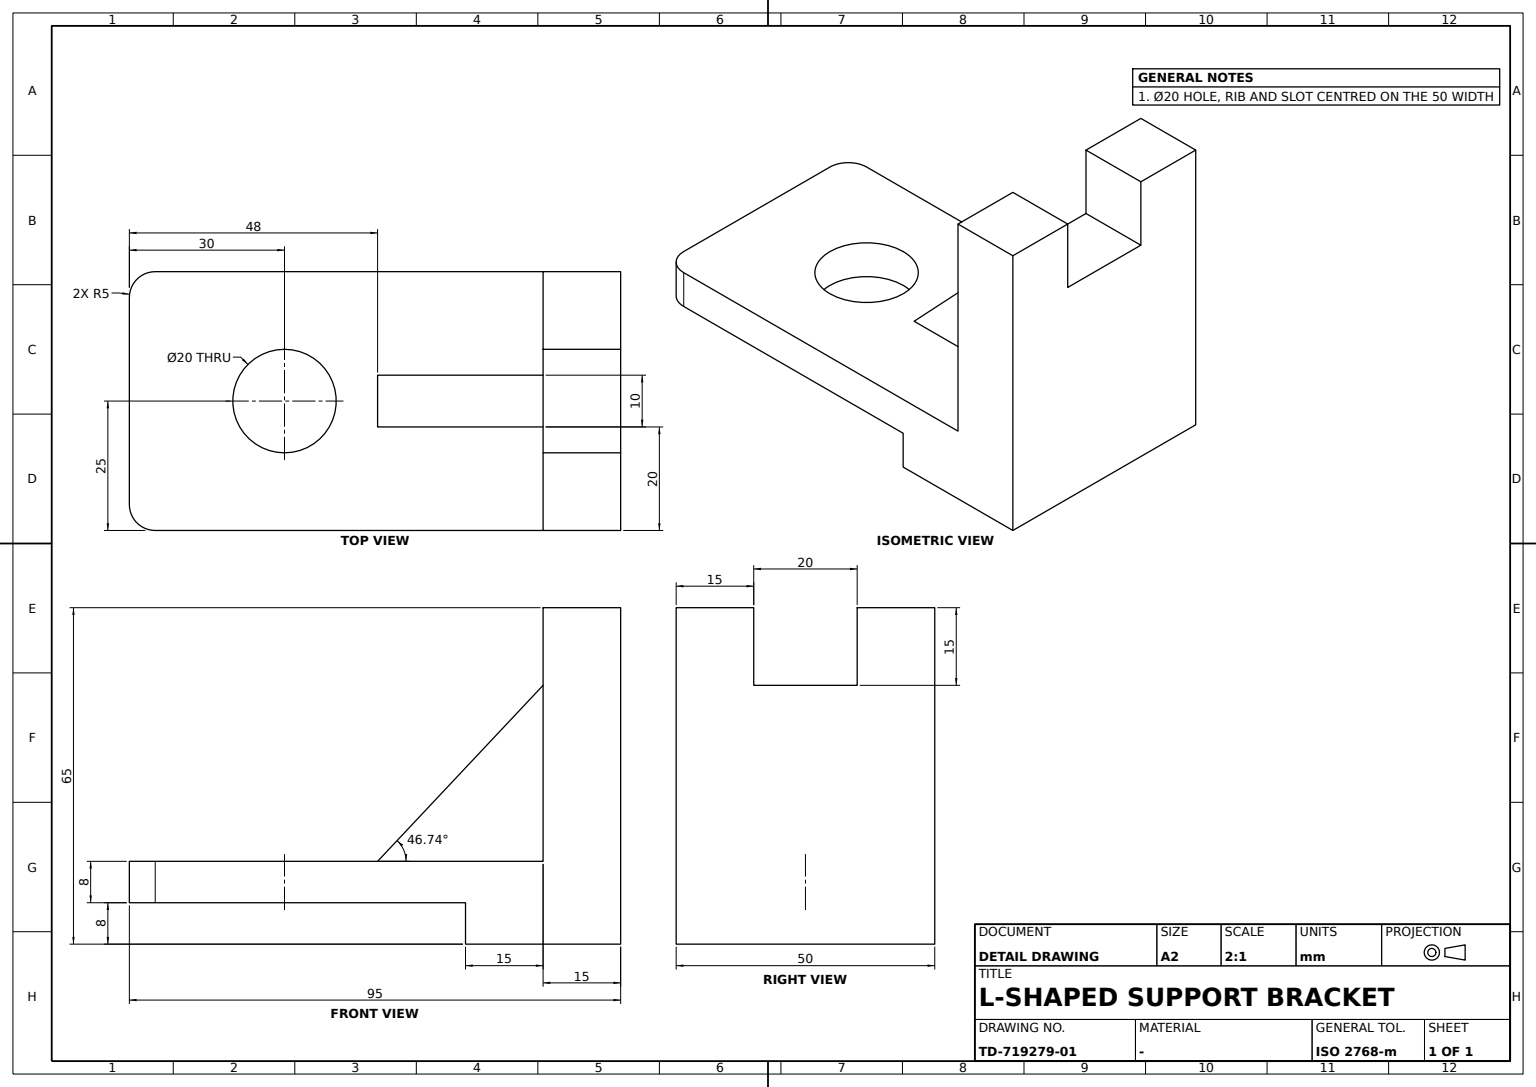
ISO-10303-21;
HEADER;
FILE_DESCRIPTION((''),'2;1');
FILE_NAME('','',(''),(''),'','','');
FILE_SCHEMA(('AUTOMOTIVE_DESIGN'));
ENDSEC;
DATA;
#1=APPLICATION_CONTEXT('');
#2=PRODUCT_CONTEXT('',#1,'mechanical');
#3=PRODUCT('','','',(#2));
#4=PRODUCT_DEFINITION_FORMATION('','',#3);
#5=PRODUCT_DEFINITION_CONTEXT('',#1,'design');
#6=PRODUCT_DEFINITION('','',#4,#5);
#7=PRODUCT_DEFINITION_SHAPE('','',#6);
#8=(LENGTH_UNIT()NAMED_UNIT(*)SI_UNIT(.MILLI.,.METRE.));
#9=(NAMED_UNIT(*)PLANE_ANGLE_UNIT()SI_UNIT($,.RADIAN.));
#10=(NAMED_UNIT(*)SI_UNIT($,.STERADIAN.)SOLID_ANGLE_UNIT());
#11=UNCERTAINTY_MEASURE_WITH_UNIT(LENGTH_MEASURE(0.005),#8,'distance_accuracy_value','');
#12=(GEOMETRIC_REPRESENTATION_CONTEXT(3)GLOBAL_UNCERTAINTY_ASSIGNED_CONTEXT((#11))GLOBAL_UNIT_ASSIGNED_CONTEXT((#8,#9,#10))REPRESENTATION_CONTEXT('',''));
#13=CARTESIAN_POINT('',(-5.,-47.,16.));
#14=VERTEX_POINT('',#13);
#15=CARTESIAN_POINT('',(-5.,-15.,16.));
#16=VERTEX_POINT('',#15);
#17=CARTESIAN_POINT('',(-5.,0.,16.));
#18=DIRECTION('',(0.,1.,0.));
#19=VECTOR('',#18,1000.);
#20=LINE('',#17,#19);
#21=EDGE_CURVE('',#14,#16,#20,.T.);
#22=ORIENTED_EDGE('',*,*,#21,.F.);
#23=CARTESIAN_POINT('',(-5.,-15.,50.));
#24=VERTEX_POINT('',#23);
#25=DIRECTION('',(0.,0.685364699,0.728199993));
#26=VECTOR('',#25,1000.);
#27=LINE('',#13,#26);
#28=EDGE_CURVE('',#14,#24,#27,.T.);
#29=ORIENTED_EDGE('',*,*,#28,.T.);
#30=CARTESIAN_POINT('',(-5.,-15.,0.));
#31=DIRECTION('',(0.,0.,1.));
#32=VECTOR('',#31,1000.);
#33=LINE('',#30,#32);
#34=EDGE_CURVE('',#16,#24,#33,.T.);
#35=ORIENTED_EDGE('',*,*,#34,.F.);
#36=EDGE_LOOP('',(#22,#29,#35));
#37=FACE_BOUND('',#36,.T.);
#38=CARTESIAN_POINT('',(-5.,0.,0.));
#39=DIRECTION('',(-1.,0.,0.));
#40=AXIS2_PLACEMENT_3D('',#38,#39,#31);
#41=PLANE('',#40);
#42=ADVANCED_FACE('',(#37),#41,.T.);
#43=CARTESIAN_POINT('',(20.,-95.,8.));
#44=VERTEX_POINT('',#43);
#45=CARTESIAN_POINT('',(-20.,-95.,8.));
#46=VERTEX_POINT('',#45);
#47=CARTESIAN_POINT('',(25.,-95.,8.));
#48=VECTOR('',#39,1000.);
#49=LINE('',#47,#48);
#50=EDGE_CURVE('',#44,#46,#49,.T.);
#51=ORIENTED_EDGE('',*,*,#50,.F.);
#52=CARTESIAN_POINT('',(20.,-95.,16.));
#53=VERTEX_POINT('',#52);
#54=LINE('',#52,#32);
#55=EDGE_CURVE('',#44,#53,#54,.T.);
#56=ORIENTED_EDGE('',*,*,#55,.T.);
#57=CARTESIAN_POINT('',(-20.,-95.,16.));
#58=VERTEX_POINT('',#57);
#59=CARTESIAN_POINT('',(25.,-95.,16.));
#60=LINE('',#59,#48);
#61=EDGE_CURVE('',#53,#58,#60,.T.);
#62=ORIENTED_EDGE('',*,*,#61,.T.);
#63=DIRECTION('',(0.,0.,-1.));
#64=VECTOR('',#63,1000.);
#65=LINE('',#57,#64);
#66=EDGE_CURVE('',#58,#46,#65,.T.);
#67=ORIENTED_EDGE('',*,*,#66,.T.);
#68=EDGE_LOOP('',(#51,#56,#62,#67));
#69=FACE_BOUND('',#68,.T.);
#70=AXIS2_PLACEMENT_3D('',#59,#18,#31);
#71=PLANE('',#70);
#72=ADVANCED_FACE('',(#69),#71,.F.);
#73=CARTESIAN_POINT('',(-25.,0.,65.));
#74=VERTEX_POINT('',#73);
#75=CARTESIAN_POINT('',(-25.,-15.,65.));
#76=VERTEX_POINT('',#75);
#77=DIRECTION('',(0.,-1.,0.));
#78=VECTOR('',#77,1000.);
#79=LINE('',#73,#78);
#80=EDGE_CURVE('',#74,#76,#79,.T.);
#81=ORIENTED_EDGE('',*,*,#80,.T.);
#82=CARTESIAN_POINT('',(-10.,-15.,65.));
#83=VERTEX_POINT('',#82);
#84=CARTESIAN_POINT('',(25.,-15.,65.));
#85=LINE('',#84,#48);
#86=EDGE_CURVE('',#83,#76,#85,.T.);
#87=ORIENTED_EDGE('',*,*,#86,.F.);
#88=CARTESIAN_POINT('',(-10.,0.,65.));
#89=VERTEX_POINT('',#88);
#90=CARTESIAN_POINT('',(-10.,35.,65.));
#91=LINE('',#90,#78);
#92=EDGE_CURVE('',#89,#83,#91,.T.);
#93=ORIENTED_EDGE('',*,*,#92,.F.);
#94=CARTESIAN_POINT('',(25.,0.,65.));
#95=LINE('',#94,#48);
#96=EDGE_CURVE('',#89,#74,#95,.T.);
#97=ORIENTED_EDGE('',*,*,#96,.T.);
#98=EDGE_LOOP('',(#81,#87,#93,#97));
#99=FACE_BOUND('',#98,.T.);
#100=AXIS2_PLACEMENT_3D('',#94,#63,#18);
#101=PLANE('',#100);
#102=ADVANCED_FACE('',(#99),#101,.F.);
#103=VERTEX_POINT('',#94);
#104=VERTEX_POINT('',#84);
#105=LINE('',#94,#78);
#106=EDGE_CURVE('',#103,#104,#105,.T.);
#107=ORIENTED_EDGE('',*,*,#106,.F.);
#108=CARTESIAN_POINT('',(10.,0.,65.));
#109=VERTEX_POINT('',#108);
#110=EDGE_CURVE('',#103,#109,#95,.T.);
#111=ORIENTED_EDGE('',*,*,#110,.T.);
#112=CARTESIAN_POINT('',(10.,-15.,65.));
#113=VERTEX_POINT('',#112);
#114=CARTESIAN_POINT('',(10.,35.,65.));
#115=LINE('',#114,#78);
#116=EDGE_CURVE('',#109,#113,#115,.T.);
#117=ORIENTED_EDGE('',*,*,#116,.T.);
#118=EDGE_CURVE('',#104,#113,#85,.T.);
#119=ORIENTED_EDGE('',*,*,#118,.F.);
#120=EDGE_LOOP('',(#107,#111,#117,#119));
#121=FACE_BOUND('',#120,.T.);
#122=ADVANCED_FACE('',(#121),#101,.F.);
#123=ORIENTED_EDGE('',*,*,#28,.F.);
#124=CARTESIAN_POINT('',(5.,-47.,16.));
#125=VERTEX_POINT('',#124);
#126=LINE('',#124,#48);
#127=EDGE_CURVE('',#125,#14,#126,.T.);
#128=ORIENTED_EDGE('',*,*,#127,.F.);
#129=CARTESIAN_POINT('',(5.,-15.,50.));
#130=VERTEX_POINT('',#129);
#131=LINE('',#124,#26);
#132=EDGE_CURVE('',#125,#130,#131,.T.);
#133=ORIENTED_EDGE('',*,*,#132,.T.);
#134=LINE('',#129,#48);
#135=EDGE_CURVE('',#130,#24,#134,.T.);
#136=ORIENTED_EDGE('',*,*,#135,.T.);
#137=EDGE_LOOP('',(#123,#128,#133,#136));
#138=FACE_BOUND('',#137,.T.);
#139=DIRECTION('',(0.,-0.728199993,0.685364699));
#140=DIRECTION('',(0.,-0.685364699,-0.728199993));
#141=AXIS2_PLACEMENT_3D('',#124,#139,#140);
#142=PLANE('',#141);
#143=ADVANCED_FACE('',(#138),#142,.T.);
#144=CARTESIAN_POINT('',(-25.,-90.,16.));
#145=VERTEX_POINT('',#144);
#146=CARTESIAN_POINT('',(-20.,-90.,16.));
#147=AXIS2_PLACEMENT_3D('',#146,#31,#39);
#148=CIRCLE('',#147,5.);
#149=EDGE_CURVE('',#145,#58,#148,.T.);
#150=ORIENTED_EDGE('',*,*,#149,.F.);
#151=CARTESIAN_POINT('',(-25.,-90.,8.));
#152=VERTEX_POINT('',#151);
#153=CARTESIAN_POINT('',(-25.,-90.,0.));
#154=LINE('',#153,#32);
#155=EDGE_CURVE('',#152,#145,#154,.T.);
#156=ORIENTED_EDGE('',*,*,#155,.F.);
#157=CARTESIAN_POINT('',(-20.,-90.,8.));
#158=AXIS2_PLACEMENT_3D('',#157,#63,#77);
#159=CIRCLE('',#158,5.);
#160=EDGE_CURVE('',#46,#152,#159,.T.);
#161=ORIENTED_EDGE('',*,*,#160,.F.);
#162=ORIENTED_EDGE('',*,*,#66,.F.);
#163=EDGE_LOOP('',(#150,#156,#161,#162));
#164=FACE_BOUND('',#163,.T.);
#165=AXIS2_PLACEMENT_3D('',#146,#63,#18);
#166=CYLINDRICAL_SURFACE('',#165,5.);
#167=ADVANCED_FACE('',(#164),#166,.T.);
#168=CARTESIAN_POINT('',(10.,-15.,50.));
#169=VERTEX_POINT('',#168);
#170=CARTESIAN_POINT('',(-10.,-15.,50.));
#171=DIRECTION('',(1.,0.,0.));
#172=VECTOR('',#171,1000.);
#173=LINE('',#170,#172);
#174=EDGE_CURVE('',#130,#169,#173,.T.);
#175=ORIENTED_EDGE('',*,*,#174,.F.);
#176=CARTESIAN_POINT('',(5.,-15.,16.));
#177=VERTEX_POINT('',#176);
#178=CARTESIAN_POINT('',(5.,-15.,0.));
#179=LINE('',#178,#64);
#180=EDGE_CURVE('',#130,#177,#179,.T.);
#181=ORIENTED_EDGE('',*,*,#180,.T.);
#182=CARTESIAN_POINT('',(25.,-15.,16.));
#183=VERTEX_POINT('',#182);
#184=LINE('',#182,#48);
#185=EDGE_CURVE('',#183,#177,#184,.T.);
#186=ORIENTED_EDGE('',*,*,#185,.F.);
#187=LINE('',#84,#64);
#188=EDGE_CURVE('',#104,#183,#187,.T.);
#189=ORIENTED_EDGE('',*,*,#188,.F.);
#190=ORIENTED_EDGE('',*,*,#118,.T.);
#191=LINE('',#168,#32);
#192=EDGE_CURVE('',#169,#113,#191,.T.);
#193=ORIENTED_EDGE('',*,*,#192,.F.);
#194=EDGE_LOOP('',(#175,#181,#186,#189,#190,#193));
#195=FACE_BOUND('',#194,.T.);
#196=AXIS2_PLACEMENT_3D('',#84,#18,#31);
#197=PLANE('',#196);
#198=ADVANCED_FACE('',(#195),#197,.F.);
#199=CARTESIAN_POINT('',(10.,-65.,16.));
#200=VERTEX_POINT('',#199);
#201=CARTESIAN_POINT('',(-10.,-65.,16.));
#202=VERTEX_POINT('',#201);
#203=CARTESIAN_POINT('',(0.,-65.,16.));
#204=AXIS2_PLACEMENT_3D('',#203,#31,#171);
#205=CIRCLE('',#204,10.);
#206=EDGE_CURVE('',#200,#202,#205,.T.);
#207=ORIENTED_EDGE('',*,*,#206,.F.);
#208=EDGE_CURVE('',#202,#200,#205,.T.);
#209=ORIENTED_EDGE('',*,*,#208,.F.);
#210=EDGE_LOOP('',(#207,#209));
#211=FACE_BOUND('',#210,.T.);
#212=CARTESIAN_POINT('',(5.,0.,16.));
#213=LINE('',#212,#78);
#214=EDGE_CURVE('',#177,#125,#213,.T.);
#215=ORIENTED_EDGE('',*,*,#214,.T.);
#216=ORIENTED_EDGE('',*,*,#127,.T.);
#217=ORIENTED_EDGE('',*,*,#21,.T.);
#218=CARTESIAN_POINT('',(-25.,-15.,16.));
#219=VERTEX_POINT('',#218);
#220=EDGE_CURVE('',#16,#219,#184,.T.);
#221=ORIENTED_EDGE('',*,*,#220,.T.);
#222=LINE('',#218,#78);
#223=EDGE_CURVE('',#219,#145,#222,.T.);
#224=ORIENTED_EDGE('',*,*,#223,.T.);
#225=ORIENTED_EDGE('',*,*,#149,.T.);
#226=ORIENTED_EDGE('',*,*,#61,.F.);
#227=CARTESIAN_POINT('',(25.,-90.,16.));
#228=VERTEX_POINT('',#227);
#229=CARTESIAN_POINT('',(20.,-90.,16.));
#230=AXIS2_PLACEMENT_3D('',#229,#31,#39);
#231=CIRCLE('',#230,5.);
#232=EDGE_CURVE('',#53,#228,#231,.T.);
#233=ORIENTED_EDGE('',*,*,#232,.T.);
#234=LINE('',#182,#78);
#235=EDGE_CURVE('',#183,#228,#234,.T.);
#236=ORIENTED_EDGE('',*,*,#235,.F.);
#237=ORIENTED_EDGE('',*,*,#185,.T.);
#238=EDGE_LOOP('',(#215,#216,#217,#221,#224,#225,#226,#233,#236,#237));
#239=FACE_BOUND('',#238,.T.);
#240=AXIS2_PLACEMENT_3D('',#182,#63,#39);
#241=PLANE('',#240);
#242=ADVANCED_FACE('',(#211,#239),#241,.F.);
#243=ORIENTED_EDGE('',*,*,#180,.F.);
#244=ORIENTED_EDGE('',*,*,#132,.F.);
#245=ORIENTED_EDGE('',*,*,#214,.F.);
#246=EDGE_LOOP('',(#243,#244,#245));
#247=FACE_BOUND('',#246,.T.);
#248=CARTESIAN_POINT('',(5.,0.,0.));
#249=AXIS2_PLACEMENT_3D('',#248,#39,#31);
#250=PLANE('',#249);
#251=ADVANCED_FACE('',(#247),#250,.F.);
#252=VERTEX_POINT('',#170);
#253=EDGE_CURVE('',#252,#24,#173,.T.);
#254=ORIENTED_EDGE('',*,*,#253,.T.);
#255=ORIENTED_EDGE('',*,*,#135,.F.);
#256=ORIENTED_EDGE('',*,*,#174,.T.);
#257=CARTESIAN_POINT('',(10.,0.,50.));
#258=VERTEX_POINT('',#257);
#259=CARTESIAN_POINT('',(10.,35.,50.));
#260=LINE('',#259,#19);
#261=EDGE_CURVE('',#169,#258,#260,.T.);
#262=ORIENTED_EDGE('',*,*,#261,.T.);
#263=CARTESIAN_POINT('',(-10.,0.,50.));
#264=VERTEX_POINT('',#263);
#265=CARTESIAN_POINT('',(25.,0.,50.));
#266=LINE('',#265,#172);
#267=EDGE_CURVE('',#264,#258,#266,.T.);
#268=ORIENTED_EDGE('',*,*,#267,.F.);
#269=CARTESIAN_POINT('',(-10.,35.,50.));
#270=LINE('',#269,#19);
#271=EDGE_CURVE('',#252,#264,#270,.T.);
#272=ORIENTED_EDGE('',*,*,#271,.F.);
#273=EDGE_LOOP('',(#254,#255,#256,#262,#268,#272));
#274=FACE_BOUND('',#273,.T.);
#275=AXIS2_PLACEMENT_3D('',#269,#63,#39);
#276=PLANE('',#275);
#277=ADVANCED_FACE('',(#274),#276,.F.);
#278=CARTESIAN_POINT('',(25.,-30.,0.));
#279=VERTEX_POINT('',#278);
#280=CARTESIAN_POINT('',(-25.,-30.,0.));
#281=VERTEX_POINT('',#280);
#282=LINE('',#278,#48);
#283=EDGE_CURVE('',#279,#281,#282,.T.);
#284=ORIENTED_EDGE('',*,*,#283,.F.);
#285=CARTESIAN_POINT('',(25.,-30.,8.));
#286=VERTEX_POINT('',#285);
#287=LINE('',#285,#64);
#288=EDGE_CURVE('',#286,#279,#287,.T.);
#289=ORIENTED_EDGE('',*,*,#288,.F.);
#290=CARTESIAN_POINT('',(-25.,-30.,8.));
#291=VERTEX_POINT('',#290);
#292=LINE('',#285,#48);
#293=EDGE_CURVE('',#286,#291,#292,.T.);
#294=ORIENTED_EDGE('',*,*,#293,.T.);
#295=LINE('',#290,#64);
#296=EDGE_CURVE('',#291,#281,#295,.T.);
#297=ORIENTED_EDGE('',*,*,#296,.T.);
#298=EDGE_LOOP('',(#284,#289,#294,#297));
#299=FACE_BOUND('',#298,.T.);
#300=AXIS2_PLACEMENT_3D('',#285,#18,#31);
#301=PLANE('',#300);
#302=ADVANCED_FACE('',(#299),#301,.F.);
#303=LINE('',#82,#64);
#304=EDGE_CURVE('',#83,#252,#303,.T.);
#305=ORIENTED_EDGE('',*,*,#304,.T.);
#306=ORIENTED_EDGE('',*,*,#271,.T.);
#307=CARTESIAN_POINT('',(-10.,0.,0.));
#308=LINE('',#307,#64);
#309=EDGE_CURVE('',#89,#264,#308,.T.);
#310=ORIENTED_EDGE('',*,*,#309,.F.);
#311=ORIENTED_EDGE('',*,*,#92,.T.);
#312=EDGE_LOOP('',(#305,#306,#310,#311));
#313=FACE_BOUND('',#312,.T.);
#314=AXIS2_PLACEMENT_3D('',#90,#39,#31);
#315=PLANE('',#314);
#316=ADVANCED_FACE('',(#313),#315,.F.);
#317=CARTESIAN_POINT('',(25.,0.,0.));
#318=VERTEX_POINT('',#317);
#319=LINE('',#317,#32);
#320=EDGE_CURVE('',#318,#103,#319,.T.);
#321=ORIENTED_EDGE('',*,*,#320,.F.);
#322=CARTESIAN_POINT('',(-25.,0.,0.));
#323=VERTEX_POINT('',#322);
#324=LINE('',#317,#48);
#325=EDGE_CURVE('',#318,#323,#324,.T.);
#326=ORIENTED_EDGE('',*,*,#325,.T.);
#327=LINE('',#322,#32);
#328=EDGE_CURVE('',#323,#74,#327,.T.);
#329=ORIENTED_EDGE('',*,*,#328,.T.);
#330=ORIENTED_EDGE('',*,*,#96,.F.);
#331=ORIENTED_EDGE('',*,*,#309,.T.);
#332=ORIENTED_EDGE('',*,*,#267,.T.);
#333=CARTESIAN_POINT('',(10.,0.,0.));
#334=LINE('',#333,#32);
#335=EDGE_CURVE('',#258,#109,#334,.T.);
#336=ORIENTED_EDGE('',*,*,#335,.T.);
#337=ORIENTED_EDGE('',*,*,#110,.F.);
#338=EDGE_LOOP('',(#321,#326,#329,#330,#331,#332,#336,#337));
#339=FACE_BOUND('',#338,.T.);
#340=AXIS2_PLACEMENT_3D('',#317,#77,#63);
#341=PLANE('',#340);
#342=ADVANCED_FACE('',(#339),#341,.F.);
#343=LINE('',#75,#64);
#344=EDGE_CURVE('',#76,#219,#343,.T.);
#345=ORIENTED_EDGE('',*,*,#344,.F.);
#346=ORIENTED_EDGE('',*,*,#80,.F.);
#347=ORIENTED_EDGE('',*,*,#328,.F.);
#348=LINE('',#280,#19);
#349=EDGE_CURVE('',#281,#323,#348,.T.);
#350=ORIENTED_EDGE('',*,*,#349,.F.);
#351=ORIENTED_EDGE('',*,*,#296,.F.);
#352=CARTESIAN_POINT('',(-25.,-95.,8.));
#353=LINE('',#352,#19);
#354=EDGE_CURVE('',#152,#291,#353,.T.);
#355=ORIENTED_EDGE('',*,*,#354,.F.);
#356=ORIENTED_EDGE('',*,*,#155,.T.);
#357=ORIENTED_EDGE('',*,*,#223,.F.);
#358=EDGE_LOOP('',(#345,#346,#347,#350,#351,#355,#356,#357));
#359=FACE_BOUND('',#358,.T.);
#360=AXIS2_PLACEMENT_3D('',#322,#171,#63);
#361=PLANE('',#360);
#362=ADVANCED_FACE('',(#359),#361,.F.);
#363=ORIENTED_EDGE('',*,*,#344,.T.);
#364=ORIENTED_EDGE('',*,*,#220,.F.);
#365=ORIENTED_EDGE('',*,*,#34,.T.);
#366=ORIENTED_EDGE('',*,*,#253,.F.);
#367=ORIENTED_EDGE('',*,*,#304,.F.);
#368=ORIENTED_EDGE('',*,*,#86,.T.);
#369=EDGE_LOOP('',(#363,#364,#365,#366,#367,#368));
#370=FACE_BOUND('',#369,.T.);
#371=ADVANCED_FACE('',(#370),#197,.F.);
#372=CARTESIAN_POINT('',(25.,-90.,8.));
#373=VERTEX_POINT('',#372);
#374=LINE('',#372,#64);
#375=EDGE_CURVE('',#228,#373,#374,.T.);
#376=ORIENTED_EDGE('',*,*,#375,.F.);
#377=ORIENTED_EDGE('',*,*,#232,.F.);
#378=ORIENTED_EDGE('',*,*,#55,.F.);
#379=CARTESIAN_POINT('',(20.,-90.,8.));
#380=AXIS2_PLACEMENT_3D('',#379,#63,#77);
#381=CIRCLE('',#380,5.);
#382=EDGE_CURVE('',#373,#44,#381,.T.);
#383=ORIENTED_EDGE('',*,*,#382,.F.);
#384=EDGE_LOOP('',(#376,#377,#378,#383));
#385=FACE_BOUND('',#384,.T.);
#386=CARTESIAN_POINT('',(20.,-90.,0.));
#387=AXIS2_PLACEMENT_3D('',#386,#31,#77);
#388=CYLINDRICAL_SURFACE('',#387,5.);
#389=ADVANCED_FACE('',(#385),#388,.T.);
#390=ORIENTED_EDGE('',*,*,#206,.T.);
#391=CARTESIAN_POINT('',(-10.,-65.,8.));
#392=VERTEX_POINT('',#391);
#393=CARTESIAN_POINT('',(-10.,-65.,-34.));
#394=LINE('',#393,#32);
#395=EDGE_CURVE('',#392,#202,#394,.T.);
#396=ORIENTED_EDGE('',*,*,#395,.F.);
#397=CARTESIAN_POINT('',(10.,-65.,8.));
#398=VERTEX_POINT('',#397);
#399=CARTESIAN_POINT('',(0.,-65.,8.));
#400=AXIS2_PLACEMENT_3D('',#399,#31,#77);
#401=CIRCLE('',#400,10.);
#402=EDGE_CURVE('',#398,#392,#401,.T.);
#403=ORIENTED_EDGE('',*,*,#402,.F.);
#404=CARTESIAN_POINT('',(10.,-65.,-34.));
#405=LINE('',#404,#32);
#406=EDGE_CURVE('',#200,#398,#405,.F.);
#407=ORIENTED_EDGE('',*,*,#406,.F.);
#408=EDGE_LOOP('',(#390,#396,#403,#407));
#409=FACE_BOUND('',#408,.T.);
#410=CARTESIAN_POINT('',(0.,-65.,-34.));
#411=AXIS2_PLACEMENT_3D('',#410,#31,#171);
#412=CYLINDRICAL_SURFACE('',#411,10.);
#413=ADVANCED_FACE('',(#409),#412,.F.);
#414=ORIENTED_EDGE('',*,*,#406,.T.);
#415=EDGE_CURVE('',#392,#398,#401,.T.);
#416=ORIENTED_EDGE('',*,*,#415,.F.);
#417=ORIENTED_EDGE('',*,*,#395,.T.);
#418=ORIENTED_EDGE('',*,*,#208,.T.);
#419=EDGE_LOOP('',(#414,#416,#417,#418));
#420=FACE_BOUND('',#419,.T.);
#421=ADVANCED_FACE('',(#420),#412,.F.);
#422=ORIENTED_EDGE('',*,*,#325,.F.);
#423=LINE('',#278,#19);
#424=EDGE_CURVE('',#279,#318,#423,.T.);
#425=ORIENTED_EDGE('',*,*,#424,.F.);
#426=ORIENTED_EDGE('',*,*,#283,.T.);
#427=ORIENTED_EDGE('',*,*,#349,.T.);
#428=EDGE_LOOP('',(#422,#425,#426,#427));
#429=FACE_BOUND('',#428,.T.);
#430=AXIS2_PLACEMENT_3D('',#278,#31,#77);
#431=PLANE('',#430);
#432=ADVANCED_FACE('',(#429),#431,.F.);
#433=ORIENTED_EDGE('',*,*,#293,.F.);
#434=LINE('',#47,#19);
#435=EDGE_CURVE('',#373,#286,#434,.T.);
#436=ORIENTED_EDGE('',*,*,#435,.F.);
#437=ORIENTED_EDGE('',*,*,#382,.T.);
#438=ORIENTED_EDGE('',*,*,#50,.T.);
#439=ORIENTED_EDGE('',*,*,#160,.T.);
#440=ORIENTED_EDGE('',*,*,#354,.T.);
#441=EDGE_LOOP('',(#433,#436,#437,#438,#439,#440));
#442=FACE_BOUND('',#441,.T.);
#443=ORIENTED_EDGE('',*,*,#402,.T.);
#444=ORIENTED_EDGE('',*,*,#415,.T.);
#445=EDGE_LOOP('',(#443,#444));
#446=FACE_BOUND('',#445,.T.);
#447=AXIS2_PLACEMENT_3D('',#47,#31,#77);
#448=PLANE('',#447);
#449=ADVANCED_FACE('',(#442,#446),#448,.F.);
#450=ORIENTED_EDGE('',*,*,#192,.T.);
#451=ORIENTED_EDGE('',*,*,#116,.F.);
#452=ORIENTED_EDGE('',*,*,#335,.F.);
#453=ORIENTED_EDGE('',*,*,#261,.F.);
#454=EDGE_LOOP('',(#450,#451,#452,#453));
#455=FACE_BOUND('',#454,.T.);
#456=AXIS2_PLACEMENT_3D('',#259,#171,#63);
#457=PLANE('',#456);
#458=ADVANCED_FACE('',(#455),#457,.F.);
#459=ORIENTED_EDGE('',*,*,#424,.T.);
#460=ORIENTED_EDGE('',*,*,#320,.T.);
#461=ORIENTED_EDGE('',*,*,#106,.T.);
#462=ORIENTED_EDGE('',*,*,#188,.T.);
#463=ORIENTED_EDGE('',*,*,#235,.T.);
#464=ORIENTED_EDGE('',*,*,#375,.T.);
#465=ORIENTED_EDGE('',*,*,#435,.T.);
#466=ORIENTED_EDGE('',*,*,#288,.T.);
#467=EDGE_LOOP('',(#459,#460,#461,#462,#463,#464,#465,#466));
#468=FACE_BOUND('',#467,.T.);
#469=AXIS2_PLACEMENT_3D('',#317,#171,#63);
#470=PLANE('',#469);
#471=ADVANCED_FACE('',(#468),#470,.T.);
#472=CLOSED_SHELL('',(#42,#72,#102,#122,#143,#167,#198,#242,#251,#277,#302,#316,#342,#362,#371,#389,#413,#421,#432,#449,#458,#471));
#473=MANIFOLD_SOLID_BREP('',#472);
#474=ADVANCED_BREP_SHAPE_REPRESENTATION('',(#473),#12);
#475=SHAPE_DEFINITION_REPRESENTATION(#7,#474);
ENDSEC;
END-ISO-10303-21;
